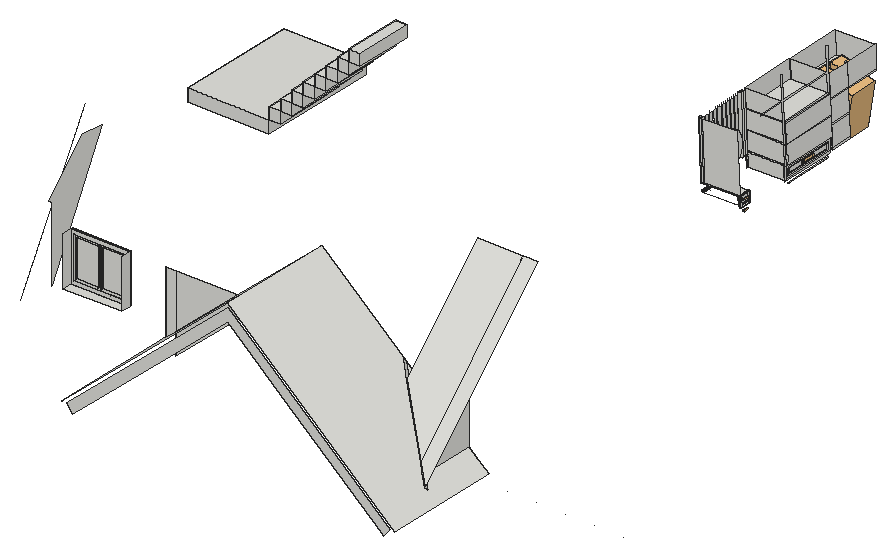
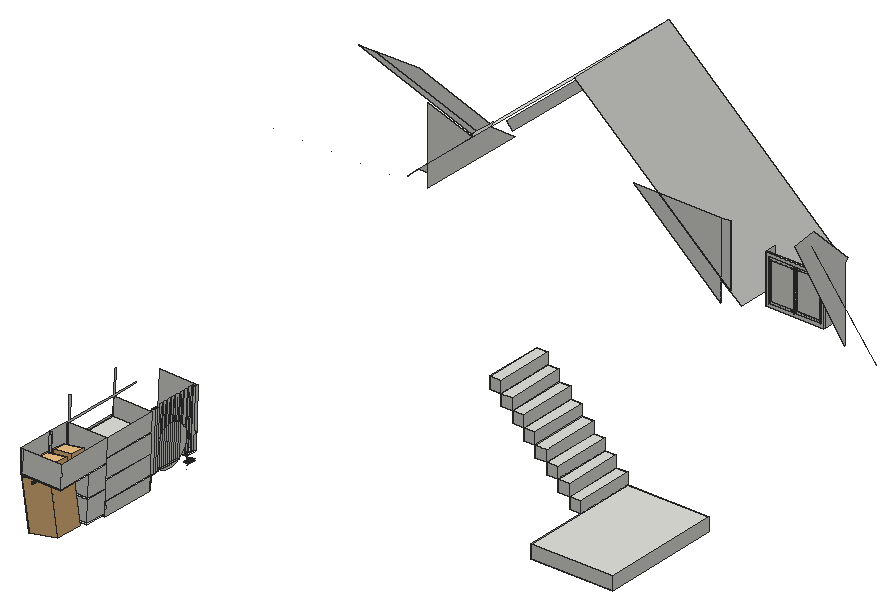
# SketchUp Ruby script. Lengths in inches.
U = 1.inch
M = Sketchup.active_model
def pt(a) = Geom::Point3d.new(a.map { |v| v * U })
def face(e, loops, mat)
  f = e.add_face(loops[0].map { |a| pt(a) })
  loops[1..].each { |l| e.add_face(l.map { |a| pt(a) }).erase! }
  f.material = f.back_material = mat if mat
  f
end
# faces: each face lists its corners as indices into pts; further lists are holes
def faces(e, pts, list, mat = nil) = list.each { |f| face(e, (f[0].is_a?(Array) ? f : [f]).map { |l| l.map { |i| pts[i] } }, mat) }
# xy, xz, yz: faces in a plane at the given z, y or x. An outline is a flat list of corners, or four numbers for a rectangle; further outlines are holes
def ring(l) = l.size == 4 ? [[l[0], l[1]], [l[2], l[1]], [l[2], l[3]], [l[0], l[3]]] : l.each_slice(2).to_a
def flat(e, list, mat, &to3) = list.each { |f| face(e, (f[0].is_a?(Array) ? f : [f]).map { |l| ring(l).map { |u, v| to3.(u, v) } }, mat) }
def xy(e, z, list, mat = nil) = flat(e, list, mat) { |x, y| [x, y, z] }
def xz(e, y, list, mat = nil) = flat(e, list, mat) { |x, z| [x, y, z] }
def yz(e, x, list, mat = nil) = flat(e, list, mat) { |y, z| [x, y, z] }
def lines(e, pts, list) = list.each { |a, b| e.add_line(pt(pts[a]), pt(pts[b])) }
# prism: a flat outline (further loops are holes) pulled along v
def prism(e, loops, v, mat = nil)
  f = face(e, loops, mat); d = Geom::Vector3d.new(v.map { |x| x * U })
  f.pushpull(f.normal.samedirection?(d) ? d.length : -d.length)
end
def box(e, o, s, mat = nil) = prism(e, [[o, [o[0] + s[0], o[1], o[2]], [o[0] + s[0], o[1] + s[1], o[2]], [o[0], o[1] + s[1], o[2]]]], [0, 0, s[2]], mat)
def at(x, y, z, deg = 0) = Geom::Transformation.translation(pt([x, y, z])) * Geom::Transformation.rotation(ORIGIN, Z_AXIS, deg.degrees)
def axes(o, x, y, z) = Geom::Transformation.new([*x, 0, *y, 0, *z, 0, *pt(o).to_a, 1])
def part(name) = M.definitions.add(name)
# library, detail: a bought-in or finely detailed component or shape, given as its bounding box
def library(name, o, s) = part(name).tap { |d| box(d.entities, o, s) }
def detail(e, o, s) = box(e.add_group.entities, o, s)
def put(e, d, t, mat = nil) = e.add_instance(d, t).tap { |i| i.material = mat if mat }
def group(e, t, mat = nil) = e.add_group.tap { |g| g.transformation = t; g.material = mat if mat }.entities
root = M.entities
c1 = library("Group\#45",[0,0,0],[1.97,1.34,1.72])
c2 = library("Group\#39",[0,0,0],[20.25,20.65,26.42])
c3 = library("glass slippers",[0.04,-7.46,0],[64.03,49.4,30.69])
c4 = library("Group\#47",[0,0,0],[1.97,1.34,1.72])
c5 = library("Agrupar\#9",[0,0,0],[56.05,55.96,70.56])
c6 = library("Agrupar\#16",[0,0,0],[78.54,37.8,62.78])
c7 = part("Sliding window")
xy(c7.entities,0,[[0,0,4.33,55.51]])
xy(c7.entities,2.76,[[0,2.76,2,27.76],[3.15,2.76,4.33,27.76],[0,27.76,0.82,52.76],[0.82,27.76,2.36,52.76],[2.36,27.76,4.33,52.76]])
xy(c7.entities,4.72,[[2,4.72,2.4,26.38],[2.76,4.72,3.15,26.38],[0.82,29.13,1.22,50.79],[1.97,29.13,2.36,50.79]])
xy(c7.entities,36.61,[[2,4.72,2.4,26.38],[2.76,4.72,3.15,26.38],[0.82,29.13,1.22,50.79],[1.97,29.13,2.36,50.79]])
xy(c7.entities,38.58,[[0,2.76,2,27.76],[3.15,2.76,4.33,27.76],[0,27.76,0.82,52.76],[0.82,27.76,2.36,52.76],[2.36,27.76,4.33,52.76]])
xy(c7.entities,41.34,[[0,0,4.33,55.51]])
xz(c7.entities,0,[[0,0,4.33,41.34]])
xz(c7.entities,2.76,[[0,2.76,2,38.58],[3.15,2.76,4.33,38.58]])
xz(c7.entities,4.72,[[2,4.72,2.4,36.61],[2.76,4.72,3.15,36.61]])
xz(c7.entities,26.38,[[2,4.72,2.4,36.61],[2.76,4.72,3.15,36.61]])
xz(c7.entities,27.76,[[0.82,2.76,2,38.58],[2,2.76,2.36,38.58],[2.36,2.76,3.15,38.58]])
xz(c7.entities,29.13,[[0.82,4.72,1.22,36.61],[1.97,4.72,2.36,36.61]])
xz(c7.entities,50.79,[[0.82,4.72,1.22,36.61],[1.97,4.72,2.36,36.61]])
xz(c7.entities,52.76,[[0,2.76,0.82,38.58],[0.82,2.76,2.36,38.58],[2.36,2.76,4.33,38.58]])
xz(c7.entities,55.51,[[0,0,4.33,41.34]])
yz(c7.entities,0,[[[0,0,55.51,41.34],[2.76,2.76,52.76,38.58]]])
yz(c7.entities,0.82,[[[27.76,2.76,52.76,38.58],[29.13,4.72,50.79,36.61]]])
yz(c7.entities,1.22,[[29.13,4.72,50.79,36.61]])
yz(c7.entities,1.97,[[29.13,4.72,50.79,36.61]])
yz(c7.entities,2,[[[2.76,2.76,27.76,38.58],[4.72,4.72,26.38,36.61]]])
yz(c7.entities,2.36,[[[27.76,2.76,52.76,38.58],[29.13,4.72,50.79,36.61]]])
yz(c7.entities,2.4,[[4.72,4.72,26.38,36.61]])
yz(c7.entities,2.76,[[4.72,4.72,26.38,36.61]])
yz(c7.entities,3.15,[[[2.76,2.76,27.76,38.58],[4.72,4.72,26.38,36.61]]])
yz(c7.entities,4.33,[[[0,0,55.51,41.34],[2.76,2.76,52.76,38.58]]])
c8 = part("Group\#7")
xy(c8.entities,7,[[0,0,7,36]])
xz(c8.entities,0,[[0,0,7,7]])
yz(c8.entities,0,[[0,0,36,7]])
yz(c8.entities,7,[[0,0,36,7]])
c9 = part("Group\#11")
xy(c9.entities,0,[[0,0,7,36]])
xz(c9.entities,36,[[0,0,7,7]])
put(c9.entities,c8,at(0,0,0))
c10 = part("Group\#15")
xy(c10.entities,0,[[0,0,7,36]])
xz(c10.entities,36,[[0,0,7,7]])
put(c10.entities,c8,at(0,0,0))
c11 = part("Group\#13")
xy(c11.entities,0,[[0,0,7,36]])
xz(c11.entities,36,[[0,0,7,7]])
put(c11.entities,c8,at(0,0,0))
c12 = part("Group\#12")
xy(c12.entities,0,[[0,0,7,36]])
xz(c12.entities,36,[[0,0,7,7]])
put(c12.entities,c8,at(0,0,0))
c13 = part("Group\#16")
xy(c13.entities,0,[[0,0,7,36]])
xz(c13.entities,36,[[0,0,7,7]])
put(c13.entities,c8,at(0,0,0))
c14 = part("Group\#9")
xy(c14.entities,0,[[0,0,7,36]])
xz(c14.entities,36,[[0,0,7,7]])
put(c14.entities,c8,at(0,0,0))
c15 = part("Group\#14")
xy(c15.entities,0,[[0,0,7,36]])
xz(c15.entities,36,[[0,0,7,7]])
put(c15.entities,c8,at(0,0,0))
c16 = part("Group\#8")
xy(c16.entities,7,[[0,0,7,36]])
xz(c16.entities,0,[[0,0,7,7]])
yz(c16.entities,0,[[0,0,36,7]])
yz(c16.entities,7,[[0,0,36,7]])
c17 = library("Group\#48",[0,0,0],[7.43,5.95,5.02])
c18 = library("Agrupar\#18",[0,0,0],[12.47,6.48,8.13])
c19 = library("Agrupar\#22",[0,-0.07,0],[12.15,18.33,3.81])
c20 = library("Agrupar\#10",[0,-0.07,0],[12.15,18.33,3.81])
xy(root,180,[[122,73.565,158,79.565]])
xz(root,1.565,[[185.31,164.988,189.605,168.749,243.605,216.049,281.013,248.816,318.42,215.974,372.397,168.584,376.493,164.988,380.297,169.321,281.017,256.485,181.511,169.325]])
xz(root,73.565,[[371,166.993,317.459,214,332.616,214,371,180.301],[191,167.157,191,180.451,191.068,180.51,191.068,167.216],[191.068,167.216,191.068,180.51,229.302,214,244.479,214],[185.068,175.254,185.113,175.294,185.113,214,185.068,214],[185.113,175.294,191,180.451,191,214,185.113,214],
  [371,175.307,371,180.301,376.6875,175.307],[191,180.451,191.068,180.51,191.068,214,191,214],[191.068,180.51,229.302,214,191.068,214]])
yz(root,110,[[79.565,174.507,79.565,220.016,77.662,221.914,103.579,247.898,118.313,246]])
yz(root,122,[[73.565,180,79.565,210]])
yz(root,158,[[73.565,180,79.565,210]])
yz(root,371,[[39.953,180.301,73.565,180.301,73.565,214]])
p = [[313.078,391.883,165.29],[313.078,420.615,165.942],[313.274,420.615,165.946],[313.274,391.882,165.294],[313.071,421.285,166.239],[313.071,391.594,165.565],
  [313.268,391.594,165.57],[313.268,421.284,166.244],[313.265,391.48,165.679],[313.265,421.393,166.358],[313.256,421.778,166.76],[313.256,391.077,166.064],
  [313.069,391.48,165.675],[313.069,393.054,165.71],[313.069,421.394,166.353],[313.078,421.009,165.951],[313.274,421.009,165.955],[289.774,389.479,167.07],
  [289.584,389.29,175.432],[289.584,388.502,175.414],[289.774,388.692,167.052],[289.774,423.329,167.838],[289.584,423.139,176.2],[313.201,389.448,168.463],
  [313.205,389.451,168.302],[313.212,389.458,167.995],[313.381,389.458,167.999],[313.389,389.467,167.606],[313.221,389.467,167.602],[312.806,389.278,175.959],
  [312.928,389.399,170.595],[312.962,389.433,169.096],[312.976,389.448,168.458],[313.389,388.68,167.588],[313.221,388.68,167.584],[313.381,388.671,167.981],
  [313.389,423.317,168.374],[313.381,423.308,168.767],[313.37,423.297,169.235],[313.37,389.448,168.467],[313.374,389.451,168.306],[313.389,421.105,168.324],
  [313.212,423.308,168.763],[313.201,423.297,169.231],[312.976,423.297,169.226],[312.806,423.127,176.727],[313.221,423.317,168.37],[313.271,388.562,172.802],
  [313.355,389.433,169.105],[313.321,389.399,170.604],[313.2,389.277,175.967],[313.2,388.49,175.95],[312.878,388.562,172.793],[312.928,388.612,170.577],
  [312.962,388.646,169.078],[312.976,388.661,168.44],[313.201,388.661,168.445],[313.205,388.664,168.284],[313.212,388.671,167.977],[313.031,423.127,176.732],
  [313.031,420.915,176.682],[313.031,389.278,175.964],[313.153,389.399,170.6],[313.187,389.433,169.101],[313.067,421.588,175.122],[313.17,421.691,170.583],
  [313.17,390.991,169.886],[313.067,390.888,174.425],[313.352,354.212,168.447],[313.352,360.625,168.593],[314.213,360.625,168.612],[314.213,354.211,168.467],
  [313.204,354,174.986],[313.208,354.004,174.805],[313.218,354.014,174.38],[313.338,354.134,169.084],[313.342,354.138,168.903],[312.481,354.139,168.883],
  [312.343,354.001,174.966],[313.342,360.766,169.053],[314.203,354.138,168.922],[314.203,360.765,169.073],[313.338,354.159,169.084],[313.342,360.79,169.054],
  [313.338,360.786,169.235],[313.338,354.461,169.091],[313.208,354.029,174.806],[313.208,360.657,174.956],[313.218,360.666,174.531],[313.342,360.815,169.054],
  [313.204,360.677,175.137],[313.208,353.979,174.804],[313.218,353.989,174.379],[313.338,354.109,169.083],[314.199,354.109,169.103],[314.069,353.979,174.824],
  [313.213,353.979,174.805],[313.218,354.039,174.38],[313.218,360.604,174.497],[313.327,360.713,169.69],[313.327,354.212,169.543],[313.218,354.103,174.35],
  [313.218,360.516,174.496],[314.199,360.786,169.254],[313.349,360.786,169.235],[312.477,354.16,169.065],[312.477,360.787,169.215],[314.053,360.677,175.157],
  [314.226,360.812,169.209],[314.059,360.681,174.976],[312.428,360.657,174.938],[312.4375,360.667,174.513],[312.347,360.657,174.936],[313.229,360.666,174.531],
  [313.2,423.127,176.736],[178.524,73.565,169.522],[178.524,1.565,169.522],[281.019,1.565,259.3],[281.019,73.565,259.3],[229.302,73.565,214],
  [191.068,73.565,180.51],[191,73.565,180.451],[185.113,73.565,175.294],[185.068,73.565,175.254],[376.6875,73.565,175.307],[371,73.565,180.301],
  [371,39.953,180.301],[332.616,73.565,214],[383.285,1.565,169.515],[383.285,73.565,169.515],[312.357,354.103,174.33],[312.466,354.212,169.523],
  [312.466,360.714,169.671],[312.357,360.604,174.478],[312.357,360.517,174.476],[313.318,354.071,169.472],[313.319,354.71,169.487],[313.319,354.071,169.472],
  [289.69,356.474,169.522],[289.69,355.552,169.501],[291.677,355.551,169.546],[291.677,356.473,169.567],[289.69,358.319,169.564],[289.69,357.397,169.543],
  [291.677,357.396,169.588],[291.677,358.318,169.609],[313.352,424.066,170.064],[289.736,424.078,169.528],[289.736,437.067,169.823],[313.352,437.055,170.359],
  [289.684,354.852,169.741],[289.684,354.065,169.723],[291.652,354.064,169.768],[291.652,354.851,169.786],[289.684,356.426,169.777],[289.684,355.639,169.759],
  [291.652,355.638,169.804],[291.652,356.425,169.822],[289.684,358.001,169.813],[289.684,357.214,169.795],[291.652,357.213,169.84],[291.652,358,169.857],
  [289.684,359.575,169.849],[289.684,358.788,169.831],[291.652,358.787,169.875],[291.652,359.574,169.893],[313.161,391.375,170.289],[313.076,391.29,174.041],
  [313.161,421.289,170.968],[289.679,359.571,170.051],[289.679,358.783,170.033],[291.647,358.782,170.078],[291.647,359.57,170.096],[313.334,437.037,171.146],
  [313.334,424.048,170.851],[314.532,424.065,170.091],[314.514,424.048,170.878],[314.532,437.054,170.386],[314.514,437.036,171.173],[312.964,421.289,170.963],
  [312.879,421.204,174.715],[312.879,392.865,174.072],[312.879,391.29,174.036],[312.964,391.375,170.284],[312.961,421.175,171.072],[312.961,391.484,170.398],
  [312.881,391.404,173.927],[312.881,421.095,174.601],[289.423,423.766,183.301],[289.718,424.06,170.315],[289.718,437.049,170.61],[289.423,436.754,183.595],
  [313.039,423.753,183.836],[313.2,423.914,176.754],[313.158,391.484,170.403],[313.078,391.404,173.932],[313.158,421.175,171.077],[313.078,421.095,174.606],
  [313.085,420.819,174.317],[313.152,420.886,171.352],[313.152,391.76,170.691],[313.085,391.693,173.656],[313.085,420.425,174.308],[312.806,388.49,175.941],
  [313.076,421.204,174.72],[313.039,436.742,184.131],[312.955,391.76,170.687],[312.888,391.693,173.652],[312.955,420.886,171.348],[312.888,420.819,174.313],
  [312.888,420.426,174.304],[314.38,423.914,176.78],[314.22,436.742,184.158],[314.22,423.753,183.863],[291.174,361.359,191.48],[291.23,359.841,188.992],
  [291.235,359.704,188.769],[291.305,358.794,185.679],[291.378,358.716,182.46],[291.449,359.473,179.33],[291.475,360.085,178.208],[291.514,361.015,176.502],
  [291.531,361.716,175.767],[291.568,363.237,174.17],[291.569,363.329,174.114],[291.592,364.926,173.14],[291.607,365.987,172.492],[291.611,366.519,172.336],
  [291.623,368.105,171.869],[291.63,369.077,171.583],[291.63,369.687,171.568],[291.632,371.263,171.53],[291.633,372.297,171.505],[291.63,372.836,171.635],
  [291.623,374.403,172.014],[291.617,375.428,172.262],[291.611,375.966,172.555],[291.593,377.522,173.403],[291.584,378.256,173.804],[291.567,379.07,174.579],
  [291.535,380.589,176.025],[291.534,380.612,176.062],[291.478,382.13,178.55],[291.473,382.267,178.774],[291.404,383.176,181.863],[291.331,383.255,185.083],
  [291.259,382.498,188.213],[291.233,381.886,189.335],[291.194,380.955,191.04],[291.177,380.255,191.775],[291.14,378.734,193.372],[291.139,378.642,193.428],
  [291.116,377.045,194.403],[291.101,375.984,195.05],[291.097,375.452,195.207],[291.086,373.866,195.673],[291.079,372.894,195.959],[291.078,372.284,195.974],
  [291.076,370.708,196.012],[291.075,369.674,196.038],[291.078,369.135,195.907],[291.086,367.568,195.528],[291.091,366.543,195.28],[291.097,366.005,194.987],
  [291.116,364.449,194.139],[291.124,363.715,193.738],[291.141,362.901,192.964],[291.173,361.382,191.518],[289.602,360.678,173.995],[289.655,360.732,171.634],
  [289.705,360.732,171.635],[289.602,353.884,173.841],[289.584,353.866,174.628],[291.552,353.865,174.672],[313.2,353.853,175.164],[313.218,353.871,174.377],
  [313.229,353.871,174.377],[313.219,353.871,174.377],[313.219,354.51,174.391],[313.213,360.657,174.956],[313.2,360.648,175.318],[288.78,353.062,210.043],
  [290.748,353.061,210.087],[289.584,354.653,174.646],[289.584,355.44,174.664],[288.78,354.636,210.078],[288.78,354.243,210.069],[288.78,353.849,210.061],
  [291.552,354.652,174.69],[291.552,355.439,174.708],[312.396,353.05,210.578],[290.748,354.635,210.123],[290.748,354.242,210.114],[290.748,353.848,210.105],
  [312.419,360.649,175.3],[291.552,360.659,174.827],[291.552,360.162,174.815],[289.584,360.163,174.771],[289.584,358.589,174.735],[291.552,358.588,174.78],
  [291.552,357.801,174.762],[291.552,357.013,174.744],[289.584,357.014,174.699],[290.748,357.784,210.194],[290.748,357.391,210.186],[290.748,356.997,210.177],
  [290.748,356.21,210.159],[312.347,354.03,174.786],[314.069,360.681,174.976],[291.552,361.737,174.851],[291.552,360.949,174.833],[289.584,360.66,174.782],
  [291.346,360.66,174.822],[312.343,354.352,174.974],[312.343,360.678,175.118],[376.6875,34.973,175.307],[376.6875,33.07,177.205],[371,38.051,182.198],
  [289.584,383.779,175.307],[288.78,382.976,210.721],[290.748,382.975,210.766],[291.552,383.778,175.351],[291.552,385.353,175.387],[289.584,385.354,175.342],
  [288.78,384.55,210.757],[290.748,384.549,210.802],[289.584,386.928,175.378],[288.78,386.124,210.793],[290.748,386.123,210.838],[291.552,386.927,175.423],
  [312.806,420.915,176.677],[312.708,423.423,198.396],[312.396,423.111,212.168],[312.378,423.093,212.955],[312.056,422.771,227.121],[312.056,421.984,227.103],
  [312.378,422.305,212.9375],[312.378,405.774,212.5625],[312.378,405.381,212.553],[312.378,404.987,212.544],[312.378,388.456,212.169],[312.056,388.134,226.335],
  [312.056,387.347,226.317],[312.378,387.669,212.151],[312.378,371.138,211.776],[312.396,371.155,210.989],[312.396,387.687,211.364],[313.2,420.915,176.685],
  [313.021,423.736,184.623],[312.726,423.441,197.609],[312.396,422.323,212.15],[312.646,422.573,201.133],[312.664,422.591,200.346],[312.914,422.841,189.328],
  [312.932,422.859,188.541],[313.182,423.109,177.523],[313.182,389.26,176.754],[312.932,389.01,187.772],[312.914,388.992,188.559],[312.664,388.742,199.577],
  [312.646,388.724,200.364],[312.396,388.474,211.382],[289.566,389.272,176.219],[289.316,389.022,187.237],[289.566,423.121,176.987],[289.316,422.871,188.005],
  [314.363,389.259,176.781],[314.113,389.009,187.799],[314.363,423.109,177.549],[314.113,422.858,188.567],[371,119.662,264.023],[367.771,119.662,264.023],
  [367.771,40.878,185.033],[376.6875,119.662,264.023],[340.119,65.093,209.311],[332.616,71.662,215.898],[313.021,436.724,184.918],[314.202,423.735,184.65],
  [314.202,436.724,184.945],[289.405,423.748,184.088],[289.11,423.453,197.073],[289.405,436.737,184.382],[289.11,436.442,197.368],[312.726,436.43,197.904],
  [313.907,423.44,197.636],[313.907,436.429,197.93],[340.119,119.662,264.023],[314.095,388.991,188.586],[314.095,422.841,189.354],[289.298,389.004,188.024],
  [289.048,388.754,199.042],[289.298,422.853,188.792],[289.048,422.603,199.81],[313.845,388.741,199.604],[313.845,422.591,200.372],[290.748,359.359,210.23],
  [290.748,360.933,210.266],[290.748,360.539,210.257],[290.748,360.146,210.248],[290.748,378.251,210.659],[290.748,379.826,210.695],[290.748,379.432,210.686],
  [290.748,379.039,210.677],[290.748,362.507,210.302],[290.748,364.082,210.337],[290.748,375.103,210.588],[290.748,376.677,210.623],[290.748,376.283,210.614],
  [290.748,375.89,210.605],[290.748,365.656,210.373],[290.748,367.231,210.409],[290.748,366.837,210.4],[290.748,366.443,210.391],[306.269,437.283,195.019],
  [306.269,438.07,195.037],[307.056,438.07,195.055],[307.056,437.282,195.037],[307.052,438.065,195.252],[307.052,438.014,195.257],[307.051,437.966,195.276],
  [307.051,437.925,195.306],[307.05,437.892,195.346],[307.049,437.872,195.393],[307.047,437.864,195.444],[307.046,437.869,195.495],[307.045,437.888,195.543],
  [307.044,437.918,195.584],[307.044,437.958,195.617],[307.043,438.005,195.637],[307.043,438.056,195.645],[307.039,438.052,195.842],[307.039,437.265,195.824],
  [306.265,438.066,195.234],[306.265,457.352,195.671],[307.052,457.351,195.689],[307.052,457.402,195.697],[307.051,457.449,195.718],[307.051,457.489,195.75],
  [307.05,457.52,195.792],[307.049,457.538,195.839],[307.047,457.544,195.89],[307.046,457.536,195.941],[307.045,457.515,195.988],[307.044,457.483,196.028],
  [307.044,457.442,196.059],[307.043,457.394,196.077],[307.043,457.343,196.083],[307.039,457.338,196.28],[307.056,457.356,195.493],[307.056,458.143,195.51],
  [307.039,458.125,196.297],[306.269,457.356,195.475],[306.269,458.144,195.493],[306.256,438.057,195.627],[306.251,438.052,195.824],[306.256,457.343,196.065],
  [290.748,371.954,210.516],[290.748,373.528,210.552],[290.748,373.135,210.543],[290.748,372.741,210.534],[306.251,437.265,195.806],[290.748,368.805,210.445],
  [290.748,370.379,210.48],[290.748,369.986,210.471],[290.748,369.592,210.462],[306.251,457.338,196.262],[306.251,458.126,196.28],[312.726,458.078,198.395],
  [312.726,437.217,197.922],[289.11,437.229,197.386],[289.11,458.09,197.859],[312.708,436.412,198.691],[313.889,423.422,198.423],[313.889,436.411,198.717],
  [289.092,423.435,197.86],[288.78,423.123,211.633],[288.78,457.759,212.419],[289.092,458.072,198.646],[312.708,458.06,199.182],[312.708,437.199,198.709],
  [313.907,437.216,197.948],[313.889,437.198,198.735],[313.907,458.077,198.422],[313.889,458.059,199.209],[313.577,423.11,212.195],[313.577,436.099,212.49],
  [312.396,457.747,212.954],[312.396,436.887,212.481],[312.396,436.099,212.463],[313.577,436.886,212.508],[313.577,457.747,212.981],[313.827,388.723,200.391],
  [313.827,422.573,201.159],[288.78,388.486,210.847],[289.03,388.736,199.829],[289.03,422.586,200.597],[288.78,422.335,211.615],[96.831,72.079,165.129],
  [97,121.565,252],[431.596,72.05,165.132],[431.596,72.048,165.13],[395.831,72.081,165.13],[395.831,72.079,165.129],[467.361,72.02,165.133],
  [467.361,72.015,165.13],[413.713,72.066,165.131],[413.713,72.065,165.13],[449.478,72.035,165.132],[449.478,72.032,165.13],[313.221,421.105,168.32],
  [312.481,360.816,169.035],[312.405,356.715,172.304],[312.402,356.698,172.436],[312.57,358.26,172.086],[312.567,358.253,172.251],[312.408,356.557,172.146],
  [312.412,356.558,171.981],[312.426,356.661,171.345],[312.426,356.683,171.368],[312.567,358.083,172.247],[312.57,358.084,172.082],[312.339,360.674,175.299],
  [312.412,356.734,171.985],[312.408,356.727,172.15],[312.996,421.105,168.315],[312.426,356.637,171.367],[313.158,403.125,172.301],[313.154,403.121,172.472],
  [312.405,356.563,172.301],[312.334,353.962,175.356],[312.323,353.962,175.356],[313.312,402.308,172.47],[313.312,402.309,172.47],[289.584,377.482,175.164],
  [291.552,377.481,175.208],[289.584,361.738,174.806],[288.78,360.934,210.221],[289.584,375.907,175.128],[288.78,375.104,210.543],[291.552,375.906,175.173],
  [291.348,360.661,174.74],[289.584,371.184,175.021],[291.552,371.183,175.065],[289.584,372.758,175.057],[288.78,371.955,210.471],[289.584,382.205,175.271],
  [288.78,381.401,210.686],[288.78,365.657,210.328],[289.584,366.461,174.914],[291.552,366.46,174.958],[289.584,369.61,174.985],[291.552,369.609,175.03],
  [289.584,357.802,174.717],[289.584,374.333,175.092],[288.78,373.529,210.507],[289.584,368.035,174.949],[291.552,368.034,174.994],[291.552,372.757,175.101],
  [289.584,379.056,175.199],[291.552,379.055,175.244],[291.552,374.332,175.137],[288.78,370.38,210.436],[289.584,380.63,175.235],[288.78,379.827,210.65],
  [291.552,387.711,175.441],[291.552,387.714,175.441],[312.583,358.14,171.53],[312.584,358.163,171.467],[312.574,358.091,171.917],[289.684,358.579,169.826],
  [288.78,368.806,210.4],[312.422,356.718,171.534],[312.419,356.729,171.666],[312.416,356.735,171.82],[288.78,367.232,210.364],[289.806,360.931,166.731],
  [289.755,360.931,166.73],[312.799,358.091,171.923],[312.793,358.085,172.179],[312.422,356.594,171.531],[312.424,356.615,171.43],[312.424,356.703,171.432],
  [313.329,354.071,169.473],[312.584,358.208,171.468],[312.583,358.228,171.532],[312.585,358.186,171.446],[289.679,360.358,170.069],[312.416,356.565,171.816],
  [312.574,358.26,171.921],[312.578,358.255,171.767],[288.78,376.678,210.579],[312.578,358.103,171.763],[312.581,358.12,171.631],[289.684,360.362,169.866],
  [289.702,360.878,169.091],[289.702,354.083,168.936],[312.581,358.244,171.634],[312.419,356.577,171.663],[291.57,360.677,174.04],[288.804,359.384,209.11],
  [291.652,360.361,169.911],[288.78,378.252,210.614],[289.663,360.788,173.016],[289.613,360.788,173.015],[291.647,360.357,170.113],[289.69,354.63,169.48],
  [291.677,354.629,169.525],[313.209,353.975,174.986],[313.209,360.652,175.137],[314.065,353.975,175.005],[313.262,409.723,172.584],[313.261,409.722,172.624],
  [313.092,409.403,172.514],[313.141,409.414,172.684],[313.145,409.396,172.742],[313.145,409.456,172.744],[313.262,409.875,172.588],[313.148,409.461,172.586]]
faces(root,p,[[0,1,2,3],[4,5,6,7],[8,9,10,11],[9,8,12,13,14],[1,15,16,2],[17,18,19,20],[17,21,22,18],[23,24,25,26,27,28,17,18,29,30,31,32],
  [28,27,33,34],[27,26,35,33],[36,37,38,39,40,26,27,41],[36,37,42,43,44,45,22,21,46],[47,35,26,40,39,48,49,50,51],[47,52,53,54,55,56,57,58,35],[25,24,57,58],[26,25,58,35],
  [[43,59,60,61,62,63,23,24,25,42],[64,65,66,67]],[40,26,25,24],[24,23,56,57],[39,40,24,23],[68,69,70,71],[32,31,54,55],[23,32,55,56],[39,38,43,44,32,23],
  [23,32,31,63],[39,23,63,48],[38,43,42,37],[72,73,74,75,76,77,78],[79,76,80,81],[82,75,76,79,83,84,85],[86,87,88,84,83,89,90,72,73],[91,92,93,94,95,96],
  [[84,88,97,82,85],[98,99,100,101,102]],[103,94,93,75,82,85,84,104],[105,106,84,85,82],[107,90,89,108,109],[31,30,53,54],[31,30,62,63],[48,63,62,49],[110,111,88,84,106,112],
  [88,84,104,113],[59,45,44,43],[114,59,43,38],[115,116,117,118,119,120,121,122,123],[124,125,126,127,118,117,128,129],[130,131,132,133,134],[131,130,101,100],[135,136,137],
  [132,131,100,99],[138,139,140,141],[142,143,144,145],[146,147,148,149],[150,151,152,153],[133,132,99,98],[154,155,156,157],[158,159,160,161],
  [162,163,164,165],[67,66,166,167],[66,65,168,166],[169,170,171,172],[149,173,174,146],[175,176,174,146],[177,178,176,175],[149,146,175,177],
  [[179,180,181,182,183],[184,185,186,187]],[167,166,183,182],[166,168,179,183],[188,189,190,191],[192,193,174,189,188],[173,190,189,174],[186,185,194,195],[[194,196,197,195],[198,199,200,201,202]],
  [185,184,196,194],[178,177,149,173],[30,29,203,52,53],[61,62,30,29],[61,50,49,62],[204,168,65,64],[205,191,190,173],[206,207,201,200],
  [207,206,208,209,210],[208,206,200,199],[211,176,178,212,213],[193,174,176,211],[174,173,178,176],[168,204,180,179],[184,187,197,196],[173,205,212,178],
  [209,208,199,198],[214,215,216,217,218,219,220,221,222,223,224,225,226,227,228,229,230,231,232,233,234,235,236,237,238,239,240,241,242,243,244,245,246,247,248,249,250,251,252,253,254,255,256,257,258,259,260,261,262,263,264,265,266,267],[268,269,270],[51,203,52,47],[207,210,202,201],[271,272,273,274,275],[187,186,195,197],[167,204,64,67],
  [204,167,182,181,180],[130,134,102,101],[210,209,198,202],[276,277,278,113],[274,276,113,279,280],[91,73,74,92],[86,73,74,97],[86,97,88,87],
  [97,88,278],[113,278,88],[110,87,88,111],[279,87,88,113],[272,281,282,273],[281,272,283,284,285,286,287],[283,272,273,288],[284,283,288,289],
  [290,274,273,282],[289,291,292,293,282,273,288],[294,295,296,297,298,299,300,301,302,284,289,288,273,274,280],[284,285,291,289],[299,303,304,305,306,301,300],[112,307,86,87,110],[87,86,73,91,96,95,308,109,279],[309,222,221,220,296,295,310],
  [311,297,296,295,312],[110,87,279,280,294],[90,72,78,313,314],[126,315,316,317],[318,319,320,321],[322,323,324,325],[326,327,328,329],[18,22,45,330,29],
  [[331,332,333,334,335,336,337,338,339,340,341,342,343,344,345,346,51,50,347,114,193,192,348,349],[350,351,352,353,354,355,356,357,358,359,360,361]],[61,29,330,60],[50,61,60,347],[356,362,363,357],[363,362,364,365],[355,364,362,356],[60,330,45,59],[347,60,59,114],
  [357,356,366,367],[366,368,369,367],[356,355,368,366],[192,193,211,213],[354,365,364,355],[370,371,372,317,316,373],[355,354,369,368],[127,126,317,372,374,375],
  [125,127,126],[192,188,191,205],[205,376,348,192],[213,377,348,192],[205,192,213,212],[212,378,377,213],[349,348,379,380],[380,379,381,382],
  [376,381,379,348],[378,212,205,376],[383,382,381,376],[349,348,377,384],[348,376,378,377],[384,377,378,385],[376,383,385,378],[374,372,371,386],
  [357,363,365,354],[354,357,367,369],[367,387,358,357],[357,354,353,358],[387,367,369,388],[359,358,389,390],[390,389,391,392],[353,391,389,358],
  [388,369,354,353],[359,358,387,393],[387,388,394,393],[358,353,388,387],[391,353,352,392],[395,215,214,396,397,398],[353,352,394,388],[399,251,250,249,400,401,402],
  [403,266,265,264,404],[405,254,253,252,406,407,408],[409,263,262,261,410,411,412],[413,414,415,416],[415,417,418,419,420,421,422,423,424,425,426,427,428,429,430,431,416],[414,432,417,415],[432,433,434,417],[417,434,435,436,437,438,439,440,441,442,443,444,445,446,429,428,427,426,425,424,423,422,421,420,419,418],
  [447,446,445,444,443,442,441,440,439,438,437,436,435,434,448,449,450],[451,452,449,448],[433,451,448,434],[453,454,430,429],[455,453,429,446],[456,257,256,255,457,458,459],[454,460,431,430],[461,260,259,258,462,463,464],
  [465,455,446,447],[466,465,447,450],[349,380,382,383],[467,468,469,470],[349,383,471,331],[384,472,331,349],[383,349,384,385],[385,473,472,384],
  [331,474,475,332],[476,475,474,477],[478,477,474,331,471,479],[383,468,479,471],[473,385,383,471],[478,479,468,467],[480,481,479,468],[467,468,480,482],
  [482,483,481,480],[332,331,472,484],[484,472,473,485],[331,471,473,472],[483,482,467,478],[477,478,486,476],[471,479,487,488],[471,488,485,473],
  [487,479,481,489],[483,490,489,481],[479,478,483,481],[359,390,392,352],[478,486,490,483],[393,491,360,359],[359,352,351,360],[352,359,393,394],
  [394,492,491,393],[493,494,495,496],[361,360,494,493],[351,495,494,360]])
lines(root,p,[[497,498],[499,500],[501,502],[503,504],[505,506],[507,508],[41,509],[77,510],[511,512],[513,514],[307,105],[515,516],
  [517,518],[519,520],[314,521],[92,275],[522,523],[509,524],[525,517],[526,527],[528,515],[529,530],[531,532],[523,511],
  [533,534],[535,536],[537,538],[537,539],[312,540],[541,542],[543,544],[545,546],[547,548],[548,549],[550,551],[552,300],
  [553,554],[555,556],[543,557],[558,559],[553,560],[541,561],[309,535],[562,563],[564,565],[566,567],[520,568],[158,569],
  [550,570],[571,572],[154,159],[573,522],[555,574],[575,576],[577,578],[579,580],[518,581],[582,137],[583,584],[585,583],
  [169,586],[567,585],[516,587],[588,513],[569,163],[589,588],[572,573],[533,590],[568,591],[591,592],[162,593],[594,595],
  [268,271],[584,596],[597,579],[580,525],[581,571],[596,589],[268,598],[595,135],[592,566],[297,599],[593,600],[150,155],
  [587,597],[558,601],[602,603],[586,604],[569,170],[605,606],[607,608],[96,607],[138,143],[607,609],[610,611],[612,613],
  [614,615],[610,616],[605,139],[615,617],[142,569]])
detail(root,[312.91,401.89,172.03],[0.37,1.38,0.79])
detail(root,[312.95,403.06,172.22],[0.37,7.64,0.79])
put(root,c1,axes([313.65,356.15,165.78],[0,1.35988,0.03086],[-0.00985,-0.00985,0.43408],[0.43419,-0.00022,0.00985]))
put(root,c2,axes([309.71,439.45,165.96],[0.00825,0.83518,0.04048],[-0.86,-0.00008,0.1769],[0.2196,-0.05392,1.06756]))
put(root,c3,axes([313.56,431.4,171.08],[-0.11769,0.00446,0.02019],[-0.00524,-0.1193,-0.00418],[0.02,-0.005,0.1177]))
put(root,c4,axes([313.51,356.01,172.0625],[0,1.35988,0.03086],[-0.00985,-0.00985,0.43408],[0.43419,-0.00022,0.00985]))
g1 = group(root,at(62,261.57,176))
box(g1,[-14,0,-2],[50,74,8])
put(root,c5,axes([308.03,394.99,176.77],[0.0098,0.15783,0.01243],[-0.10318,0.00549,0.01165],[0.01116,-0.00881,0.10301]))
put(root,c6,axes([308.85,404.43,177.49],[0.00699,0.11249,0.00886],[-0.11219,0.00597,0.01267],[0.01214,-0.00957,0.11199]))
put(root,c7,axes([122,80.72,180],[0,-0.26726,0],[0.64851,0,0],[0,0,0.72571]))
g2 = group(root,at(154,297.57,182,-180))
xy(g2,0,[[49,0,56,36]])
xz(g2,36,[[49,0,56,7]])
put(g2,c9,at(0,0,49))
put(g2,c10,at(14,0,35))
put(g2,c11,at(28,0,21))
put(g2,c12,at(35,0,14))
put(g2,c13,at(7,0,42))
put(g2,c14,at(42,0,7))
put(g2,c15,at(21,0,28))
put(g2,c16,at(49,0,0))
put(root,c17,axes([303,426.53,186.08],[1.1273,-0.0427,-0.19341],[0.05015,1.14276,0.04004],[0.19161,-0.04791,1.12739]))
put(root,c18,axes([304.32,405.65,188.03],[0.04264,0.68656,0.05407],[-0.68469,0.03643,0.07731],[0.07407,-0.05843,0.68352]))
put(root,c19,axes([310.13,428.39,198.32],[0.0298,0.67893,0.02379],[-0.66974,0.02537,0.11491],[0.21516,-0.0538,1.26592]))
put(root,c20,axes([310.67,440.6875,198.75],[0.0298,0.67893,0.02379],[-0.66974,0.02537,0.11491],[0.21516,-0.0538,1.26592]))
